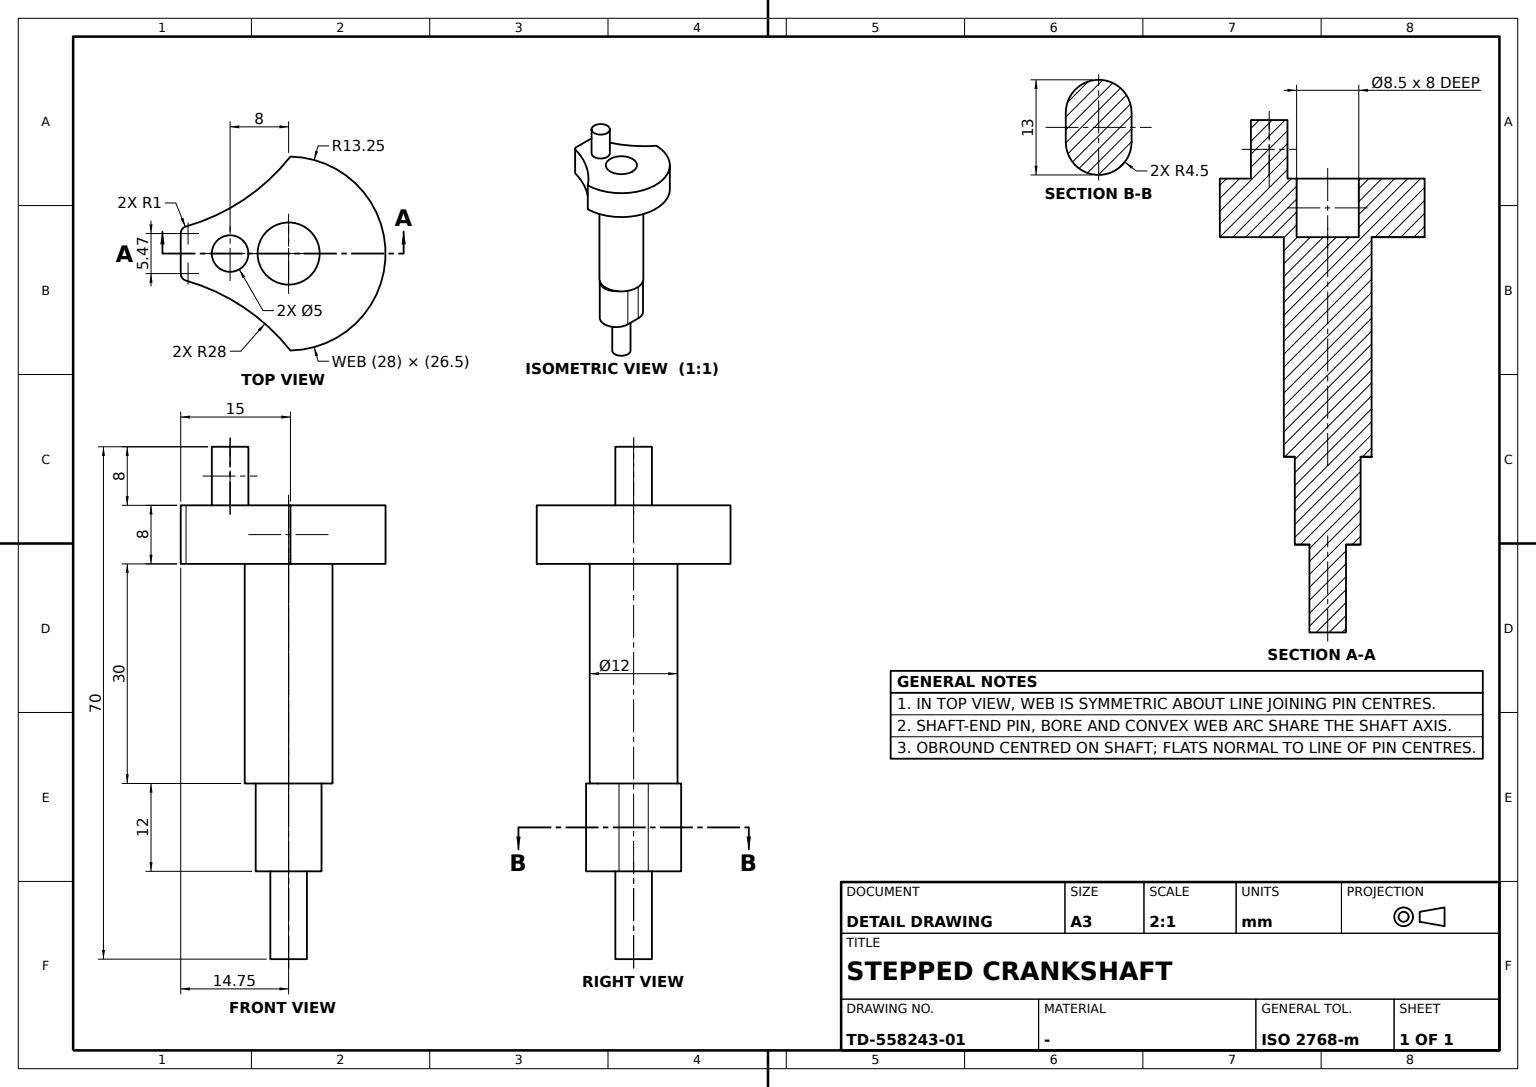
ISO-10303-21;
HEADER;
FILE_DESCRIPTION((''),'2;1');
FILE_NAME('','',(''),(''),'','','');
FILE_SCHEMA(('AUTOMOTIVE_DESIGN'));
ENDSEC;
DATA;
#1=APPLICATION_CONTEXT('');
#2=PRODUCT_CONTEXT('',#1,'mechanical');
#3=PRODUCT('','','',(#2));
#4=PRODUCT_DEFINITION_FORMATION('','',#3);
#5=PRODUCT_DEFINITION_CONTEXT('',#1,'design');
#6=PRODUCT_DEFINITION('','',#4,#5);
#7=PRODUCT_DEFINITION_SHAPE('','',#6);
#8=(LENGTH_UNIT()NAMED_UNIT(*)SI_UNIT(.MILLI.,.METRE.));
#9=(NAMED_UNIT(*)PLANE_ANGLE_UNIT()SI_UNIT($,.RADIAN.));
#10=(NAMED_UNIT(*)SI_UNIT($,.STERADIAN.)SOLID_ANGLE_UNIT());
#11=UNCERTAINTY_MEASURE_WITH_UNIT(LENGTH_MEASURE(0.005),#8,'distance_accuracy_value','');
#12=(GEOMETRIC_REPRESENTATION_CONTEXT(3)GLOBAL_UNCERTAINTY_ASSIGNED_CONTEXT((#11))GLOBAL_UNIT_ASSIGNED_CONTEXT((#8,#9,#10))REPRESENTATION_CONTEXT('',''));
#13=CARTESIAN_POINT('',(11.3410275,-4.9375,-30.));
#14=VERTEX_POINT('',#13);
#15=CARTESIAN_POINT('',(11.3410275,4.9375,-30.));
#16=VERTEX_POINT('',#15);
#17=CARTESIAN_POINT('',(14.75,0.,-30.));
#18=DIRECTION('',(0.,0.,-1.));
#19=DIRECTION('',(-1.,0.,0.));
#20=AXIS2_PLACEMENT_3D('',#17,#18,#19);
#21=CIRCLE('',#20,6.);
#22=EDGE_CURVE('',#14,#16,#21,.T.);
#23=ORIENTED_EDGE('',*,*,#22,.F.);
#24=CARTESIAN_POINT('',(18.1589725,-4.9375,-30.));
#25=VERTEX_POINT('',#24);
#26=EDGE_CURVE('',#25,#14,#21,.T.);
#27=ORIENTED_EDGE('',*,*,#26,.F.);
#28=CARTESIAN_POINT('',(18.1589725,4.9375,-30.));
#29=VERTEX_POINT('',#28);
#30=EDGE_CURVE('',#29,#25,#21,.T.);
#31=ORIENTED_EDGE('',*,*,#30,.F.);
#32=EDGE_CURVE('',#16,#29,#21,.T.);
#33=ORIENTED_EDGE('',*,*,#32,.F.);
#34=EDGE_LOOP('',(#23,#27,#31,#33));
#35=FACE_BOUND('',#34,.T.);
#36=CARTESIAN_POINT('',(20.75,0.,0.));
#37=VERTEX_POINT('',#36);
#38=CARTESIAN_POINT('',(14.75,0.,0.));
#39=DIRECTION('',(0.,0.,1.));
#40=DIRECTION('',(1.,0.,0.));
#41=AXIS2_PLACEMENT_3D('',#38,#39,#40);
#42=CIRCLE('',#41,6.);
#43=EDGE_CURVE('',#37,#37,#42,.F.);
#44=ORIENTED_EDGE('',*,*,#43,.T.);
#45=EDGE_LOOP('',(#44));
#46=FACE_BOUND('',#45,.T.);
#47=CARTESIAN_POINT('',(14.75,0.,-15.));
#48=AXIS2_PLACEMENT_3D('',#47,#18,#40);
#49=CYLINDRICAL_SURFACE('',#48,6.);
#50=ADVANCED_FACE('',(#35,#46),#49,.T.);
#51=CARTESIAN_POINT('',(19.,0.,8.));
#52=VERTEX_POINT('',#51);
#53=CARTESIAN_POINT('',(14.75,0.,8.));
#54=AXIS2_PLACEMENT_3D('',#53,#39,#40);
#55=CIRCLE('',#54,4.25);
#56=EDGE_CURVE('',#52,#52,#55,.T.);
#57=ORIENTED_EDGE('',*,*,#56,.T.);
#58=EDGE_LOOP('',(#57));
#59=FACE_BOUND('',#58,.T.);
#60=CARTESIAN_POINT('',(19.,0.,0.));
#61=VERTEX_POINT('',#60);
#62=CIRCLE('',#41,4.25);
#63=EDGE_CURVE('',#61,#61,#62,.T.);
#64=ORIENTED_EDGE('',*,*,#63,.F.);
#65=EDGE_LOOP('',(#64));
#66=FACE_BOUND('',#65,.T.);
#67=CARTESIAN_POINT('',(14.75,0.,4.));
#68=DIRECTION('',(0.,1.,0.));
#69=AXIS2_PLACEMENT_3D('',#67,#39,#68);
#70=CYLINDRICAL_SURFACE('',#69,4.25);
#71=ADVANCED_FACE('',(#59,#66),#70,.F.);
#72=CARTESIAN_POINT('',(12.25,0.,-42.));
#73=VERTEX_POINT('',#72);
#74=CARTESIAN_POINT('',(14.75,0.,-42.));
#75=AXIS2_PLACEMENT_3D('',#74,#18,#19);
#76=CIRCLE('',#75,2.5);
#77=EDGE_CURVE('',#73,#73,#76,.T.);
#78=ORIENTED_EDGE('',*,*,#77,.T.);
#79=EDGE_LOOP('',(#78));
#80=FACE_BOUND('',#79,.T.);
#81=CARTESIAN_POINT('',(12.25,0.,-54.));
#82=VERTEX_POINT('',#81);
#83=CARTESIAN_POINT('',(14.75,0.,-54.));
#84=AXIS2_PLACEMENT_3D('',#83,#18,#19);
#85=CIRCLE('',#84,2.5);
#86=EDGE_CURVE('',#82,#82,#85,.T.);
#87=ORIENTED_EDGE('',*,*,#86,.F.);
#88=EDGE_LOOP('',(#87));
#89=FACE_BOUND('',#88,.T.);
#90=CARTESIAN_POINT('',(14.75,0.,-48.));
#91=AXIS2_PLACEMENT_3D('',#90,#18,#68);
#92=CYLINDRICAL_SURFACE('',#91,2.5);
#93=ADVANCED_FACE('',(#80,#89),#92,.T.);
#94=ORIENTED_EDGE('',*,*,#63,.T.);
#95=EDGE_LOOP('',(#94));
#96=FACE_BOUND('',#95,.T.);
#97=CARTESIAN_POINT('',(0.,0.,0.));
#98=AXIS2_PLACEMENT_3D('',#97,#39,#68);
#99=PLANE('',#98);
#100=ADVANCED_FACE('',(#96),#99,.T.);
#101=CARTESIAN_POINT('',(0.7255975,3.6965592,0.));
#102=VERTEX_POINT('',#101);
#103=CARTESIAN_POINT('',(15.,13.2476413,0.));
#104=VERTEX_POINT('',#103);
#105=CARTESIAN_POINT('',(-6.9576732,30.6217769,0.));
#106=AXIS2_PLACEMENT_3D('',#105,#39,#40);
#107=CIRCLE('',#106,28.);
#108=EDGE_CURVE('',#102,#104,#107,.T.);
#109=ORIENTED_EDGE('',*,*,#108,.F.);
#110=CARTESIAN_POINT('',(0.7255975,3.6965592,8.));
#111=VERTEX_POINT('',#110);
#112=CARTESIAN_POINT('',(0.7255975,3.6965592,4.));
#113=VECTOR('',#39,1000.);
#114=LINE('',#112,#113);
#115=EDGE_CURVE('',#111,#102,#114,.F.);
#116=ORIENTED_EDGE('',*,*,#115,.F.);
#117=CARTESIAN_POINT('',(15.,13.2476413,8.));
#118=VERTEX_POINT('',#117);
#119=CARTESIAN_POINT('',(-6.9576732,30.6217769,8.));
#120=AXIS2_PLACEMENT_3D('',#119,#39,#40);
#121=CIRCLE('',#120,28.);
#122=EDGE_CURVE('',#111,#118,#121,.T.);
#123=ORIENTED_EDGE('',*,*,#122,.T.);
#124=LINE('',#103,#113);
#125=EDGE_CURVE('',#104,#118,#124,.T.);
#126=ORIENTED_EDGE('',*,*,#125,.F.);
#127=EDGE_LOOP('',(#109,#116,#123,#126));
#128=FACE_BOUND('',#127,.T.);
#129=CARTESIAN_POINT('',(-6.9576732,30.6217769,4.));
#130=AXIS2_PLACEMENT_3D('',#129,#39,#68);
#131=CYLINDRICAL_SURFACE('',#130,28.);
#132=ADVANCED_FACE('',(#128),#131,.F.);
#133=ORIENTED_EDGE('',*,*,#125,.T.);
#134=CARTESIAN_POINT('',(15.,-13.2476413,8.));
#135=VERTEX_POINT('',#134);
#136=CIRCLE('',#54,13.25);
#137=EDGE_CURVE('',#135,#118,#136,.T.);
#138=ORIENTED_EDGE('',*,*,#137,.F.);
#139=CARTESIAN_POINT('',(15.,-13.2476413,0.));
#140=VERTEX_POINT('',#139);
#141=LINE('',#139,#113);
#142=EDGE_CURVE('',#140,#135,#141,.T.);
#143=ORIENTED_EDGE('',*,*,#142,.F.);
#144=CIRCLE('',#41,13.25);
#145=EDGE_CURVE('',#140,#104,#144,.T.);
#146=ORIENTED_EDGE('',*,*,#145,.T.);
#147=EDGE_LOOP('',(#133,#138,#143,#146));
#148=FACE_BOUND('',#147,.T.);
#149=CYLINDRICAL_SURFACE('',#69,13.25);
#150=ADVANCED_FACE('',(#148),#149,.T.);
#151=ORIENTED_EDGE('',*,*,#26,.T.);
#152=CARTESIAN_POINT('',(14.75,-2.,-30.));
#153=AXIS2_PLACEMENT_3D('',#152,#18,#19);
#154=CIRCLE('',#153,4.5);
#155=EDGE_CURVE('',#25,#14,#154,.T.);
#156=ORIENTED_EDGE('',*,*,#155,.F.);
#157=EDGE_LOOP('',(#151,#156));
#158=FACE_BOUND('',#157,.T.);
#159=CARTESIAN_POINT('',(0.,0.,-30.));
#160=AXIS2_PLACEMENT_3D('',#159,#18,#40);
#161=PLANE('',#160);
#162=ADVANCED_FACE('',(#158),#161,.F.);
#163=ORIENTED_EDGE('',*,*,#43,.F.);
#164=EDGE_LOOP('',(#163));
#165=FACE_BOUND('',#164,.T.);
#166=ORIENTED_EDGE('',*,*,#108,.T.);
#167=ORIENTED_EDGE('',*,*,#145,.F.);
#168=CARTESIAN_POINT('',(0.7255975,-3.6965592,0.));
#169=VERTEX_POINT('',#168);
#170=CARTESIAN_POINT('',(-6.9576732,-30.6217769,0.));
#171=AXIS2_PLACEMENT_3D('',#170,#39,#40);
#172=CIRCLE('',#171,28.);
#173=EDGE_CURVE('',#140,#169,#172,.T.);
#174=ORIENTED_EDGE('',*,*,#173,.T.);
#175=CARTESIAN_POINT('',(0.,-2.7349442,0.));
#176=VERTEX_POINT('',#175);
#177=CARTESIAN_POINT('',(1.,-2.7349442,0.));
#178=AXIS2_PLACEMENT_3D('',#177,#39,#40);
#179=CIRCLE('',#178,1.);
#180=EDGE_CURVE('',#176,#169,#179,.T.);
#181=ORIENTED_EDGE('',*,*,#180,.F.);
#182=CARTESIAN_POINT('',(0.,2.7349442,0.));
#183=VERTEX_POINT('',#182);
#184=VECTOR('',#68,1000.);
#185=LINE('',#97,#184);
#186=EDGE_CURVE('',#176,#183,#185,.T.);
#187=ORIENTED_EDGE('',*,*,#186,.T.);
#188=CARTESIAN_POINT('',(1.,2.7349442,0.));
#189=AXIS2_PLACEMENT_3D('',#188,#39,#40);
#190=CIRCLE('',#189,1.);
#191=EDGE_CURVE('',#102,#183,#190,.T.);
#192=ORIENTED_EDGE('',*,*,#191,.F.);
#193=EDGE_LOOP('',(#166,#167,#174,#181,#187,#192));
#194=FACE_BOUND('',#193,.T.);
#195=ADVANCED_FACE('',(#165,#194),#99,.F.);
#196=CARTESIAN_POINT('',(14.75,2.,-30.));
#197=AXIS2_PLACEMENT_3D('',#196,#18,#19);
#198=CIRCLE('',#197,4.5);
#199=EDGE_CURVE('',#16,#29,#198,.T.);
#200=ORIENTED_EDGE('',*,*,#199,.F.);
#201=ORIENTED_EDGE('',*,*,#32,.T.);
#202=EDGE_LOOP('',(#200,#201));
#203=FACE_BOUND('',#202,.T.);
#204=ADVANCED_FACE('',(#203),#161,.F.);
#205=ORIENTED_EDGE('',*,*,#86,.T.);
#206=EDGE_LOOP('',(#205));
#207=FACE_BOUND('',#206,.T.);
#208=CARTESIAN_POINT('',(0.,0.,-54.));
#209=AXIS2_PLACEMENT_3D('',#208,#18,#68);
#210=PLANE('',#209);
#211=ADVANCED_FACE('',(#207),#210,.T.);
#212=CARTESIAN_POINT('',(9.25,0.,16.));
#213=VERTEX_POINT('',#212);
#214=CARTESIAN_POINT('',(6.75,0.,16.));
#215=AXIS2_PLACEMENT_3D('',#214,#39,#40);
#216=CIRCLE('',#215,2.5);
#217=EDGE_CURVE('',#213,#213,#216,.T.);
#218=ORIENTED_EDGE('',*,*,#217,.T.);
#219=EDGE_LOOP('',(#218));
#220=FACE_BOUND('',#219,.T.);
#221=CARTESIAN_POINT('',(0.,0.,16.));
#222=AXIS2_PLACEMENT_3D('',#221,#39,#40);
#223=PLANE('',#222);
#224=ADVANCED_FACE('',(#220),#223,.T.);
#225=ORIENTED_EDGE('',*,*,#56,.F.);
#226=EDGE_LOOP('',(#225));
#227=FACE_BOUND('',#226,.T.);
#228=CARTESIAN_POINT('',(0.,2.7349442,8.));
#229=VERTEX_POINT('',#228);
#230=CARTESIAN_POINT('',(1.,2.7349442,8.));
#231=AXIS2_PLACEMENT_3D('',#230,#39,#40);
#232=CIRCLE('',#231,1.);
#233=EDGE_CURVE('',#111,#229,#232,.T.);
#234=ORIENTED_EDGE('',*,*,#233,.T.);
#235=CARTESIAN_POINT('',(0.,-2.7349442,8.));
#236=VERTEX_POINT('',#235);
#237=CARTESIAN_POINT('',(0.,0.,8.));
#238=LINE('',#237,#184);
#239=EDGE_CURVE('',#236,#229,#238,.T.);
#240=ORIENTED_EDGE('',*,*,#239,.F.);
#241=CARTESIAN_POINT('',(0.7255975,-3.6965592,8.));
#242=VERTEX_POINT('',#241);
#243=CARTESIAN_POINT('',(1.,-2.7349442,8.));
#244=AXIS2_PLACEMENT_3D('',#243,#39,#40);
#245=CIRCLE('',#244,1.);
#246=EDGE_CURVE('',#236,#242,#245,.T.);
#247=ORIENTED_EDGE('',*,*,#246,.T.);
#248=CARTESIAN_POINT('',(-6.9576732,-30.6217769,8.));
#249=AXIS2_PLACEMENT_3D('',#248,#39,#40);
#250=CIRCLE('',#249,28.);
#251=EDGE_CURVE('',#135,#242,#250,.T.);
#252=ORIENTED_EDGE('',*,*,#251,.F.);
#253=ORIENTED_EDGE('',*,*,#137,.T.);
#254=ORIENTED_EDGE('',*,*,#122,.F.);
#255=EDGE_LOOP('',(#234,#240,#247,#252,#253,#254));
#256=FACE_BOUND('',#255,.T.);
#257=CARTESIAN_POINT('',(9.25,0.,8.));
#258=VERTEX_POINT('',#257);
#259=CARTESIAN_POINT('',(6.75,0.,8.));
#260=AXIS2_PLACEMENT_3D('',#259,#39,#40);
#261=CIRCLE('',#260,2.5);
#262=EDGE_CURVE('',#258,#258,#261,.T.);
#263=ORIENTED_EDGE('',*,*,#262,.F.);
#264=EDGE_LOOP('',(#263));
#265=FACE_BOUND('',#264,.T.);
#266=AXIS2_PLACEMENT_3D('',#237,#39,#68);
#267=PLANE('',#266);
#268=ADVANCED_FACE('',(#227,#256,#265),#267,.T.);
#269=ORIENTED_EDGE('',*,*,#251,.T.);
#270=CARTESIAN_POINT('',(0.7255975,-3.6965592,4.));
#271=VECTOR('',#18,1000.);
#272=LINE('',#270,#271);
#273=EDGE_CURVE('',#242,#169,#272,.T.);
#274=ORIENTED_EDGE('',*,*,#273,.T.);
#275=ORIENTED_EDGE('',*,*,#173,.F.);
#276=ORIENTED_EDGE('',*,*,#142,.T.);
#277=EDGE_LOOP('',(#269,#274,#275,#276));
#278=FACE_BOUND('',#277,.T.);
#279=CARTESIAN_POINT('',(-6.9576732,-30.6217769,4.));
#280=AXIS2_PLACEMENT_3D('',#279,#39,#68);
#281=CYLINDRICAL_SURFACE('',#280,28.);
#282=ADVANCED_FACE('',(#278),#281,.F.);
#283=CARTESIAN_POINT('',(0.,2.7349442,4.));
#284=LINE('',#283,#271);
#285=EDGE_CURVE('',#229,#183,#284,.T.);
#286=ORIENTED_EDGE('',*,*,#285,.F.);
#287=ORIENTED_EDGE('',*,*,#233,.F.);
#288=ORIENTED_EDGE('',*,*,#115,.T.);
#289=ORIENTED_EDGE('',*,*,#191,.T.);
#290=EDGE_LOOP('',(#286,#287,#288,#289));
#291=FACE_BOUND('',#290,.T.);
#292=CARTESIAN_POINT('',(1.,2.7349442,4.));
#293=AXIS2_PLACEMENT_3D('',#292,#18,#19);
#294=CYLINDRICAL_SURFACE('',#293,1.);
#295=ADVANCED_FACE('',(#291),#294,.T.);
#296=CARTESIAN_POINT('',(19.25,2.,-30.));
#297=VERTEX_POINT('',#296);
#298=CARTESIAN_POINT('',(19.25,2.,-42.));
#299=VERTEX_POINT('',#298);
#300=CARTESIAN_POINT('',(19.25,2.,-36.));
#301=LINE('',#300,#271);
#302=EDGE_CURVE('',#297,#299,#301,.T.);
#303=ORIENTED_EDGE('',*,*,#302,.F.);
#304=CARTESIAN_POINT('',(19.25,-2.,-30.));
#305=VERTEX_POINT('',#304);
#306=CARTESIAN_POINT('',(19.25,0.,-30.));
#307=LINE('',#306,#184);
#308=EDGE_CURVE('',#305,#297,#307,.T.);
#309=ORIENTED_EDGE('',*,*,#308,.F.);
#310=CARTESIAN_POINT('',(19.25,-2.,-42.));
#311=VERTEX_POINT('',#310);
#312=CARTESIAN_POINT('',(19.25,-2.,-36.));
#313=LINE('',#312,#271);
#314=EDGE_CURVE('',#305,#311,#313,.T.);
#315=ORIENTED_EDGE('',*,*,#314,.T.);
#316=CARTESIAN_POINT('',(19.25,0.,-42.));
#317=LINE('',#316,#184);
#318=EDGE_CURVE('',#311,#299,#317,.T.);
#319=ORIENTED_EDGE('',*,*,#318,.T.);
#320=EDGE_LOOP('',(#303,#309,#315,#319));
#321=FACE_BOUND('',#320,.T.);
#322=AXIS2_PLACEMENT_3D('',#304,#19,#68);
#323=PLANE('',#322);
#324=ADVANCED_FACE('',(#321),#323,.F.);
#325=ORIENTED_EDGE('',*,*,#262,.T.);
#326=EDGE_LOOP('',(#325));
#327=FACE_BOUND('',#326,.T.);
#328=ORIENTED_EDGE('',*,*,#217,.F.);
#329=EDGE_LOOP('',(#328));
#330=FACE_BOUND('',#329,.T.);
#331=CARTESIAN_POINT('',(6.75,0.,12.));
#332=AXIS2_PLACEMENT_3D('',#331,#39,#40);
#333=CYLINDRICAL_SURFACE('',#332,2.5);
#334=ADVANCED_FACE('',(#327,#330),#333,.T.);
#335=CARTESIAN_POINT('',(10.25,2.,-42.));
#336=VERTEX_POINT('',#335);
#337=CARTESIAN_POINT('',(10.25,-2.,-42.));
#338=VERTEX_POINT('',#337);
#339=CARTESIAN_POINT('',(10.25,0.,-42.));
#340=DIRECTION('',(0.,-1.,0.));
#341=VECTOR('',#340,1000.);
#342=LINE('',#339,#341);
#343=EDGE_CURVE('',#336,#338,#342,.T.);
#344=ORIENTED_EDGE('',*,*,#343,.T.);
#345=CARTESIAN_POINT('',(10.25,-2.,-30.));
#346=VERTEX_POINT('',#345);
#347=CARTESIAN_POINT('',(10.25,-2.,-36.));
#348=LINE('',#347,#271);
#349=EDGE_CURVE('',#346,#338,#348,.T.);
#350=ORIENTED_EDGE('',*,*,#349,.F.);
#351=CARTESIAN_POINT('',(10.25,2.,-30.));
#352=VERTEX_POINT('',#351);
#353=CARTESIAN_POINT('',(10.25,0.,-30.));
#354=LINE('',#353,#341);
#355=EDGE_CURVE('',#352,#346,#354,.T.);
#356=ORIENTED_EDGE('',*,*,#355,.F.);
#357=CARTESIAN_POINT('',(10.25,2.,-36.));
#358=LINE('',#357,#271);
#359=EDGE_CURVE('',#352,#336,#358,.T.);
#360=ORIENTED_EDGE('',*,*,#359,.T.);
#361=EDGE_LOOP('',(#344,#350,#356,#360));
#362=FACE_BOUND('',#361,.T.);
#363=AXIS2_PLACEMENT_3D('',#351,#40,#340);
#364=PLANE('',#363);
#365=ADVANCED_FACE('',(#362),#364,.F.);
#366=ORIENTED_EDGE('',*,*,#77,.F.);
#367=EDGE_LOOP('',(#366));
#368=FACE_BOUND('',#367,.T.);
#369=ORIENTED_EDGE('',*,*,#318,.F.);
#370=CARTESIAN_POINT('',(14.75,-2.,-42.));
#371=AXIS2_PLACEMENT_3D('',#370,#18,#19);
#372=CIRCLE('',#371,4.5);
#373=EDGE_CURVE('',#311,#338,#372,.T.);
#374=ORIENTED_EDGE('',*,*,#373,.T.);
#375=ORIENTED_EDGE('',*,*,#343,.F.);
#376=CARTESIAN_POINT('',(14.75,2.,-42.));
#377=AXIS2_PLACEMENT_3D('',#376,#18,#19);
#378=CIRCLE('',#377,4.5);
#379=EDGE_CURVE('',#336,#299,#378,.T.);
#380=ORIENTED_EDGE('',*,*,#379,.T.);
#381=EDGE_LOOP('',(#369,#374,#375,#380));
#382=FACE_BOUND('',#381,.T.);
#383=CARTESIAN_POINT('',(0.,0.,-42.));
#384=AXIS2_PLACEMENT_3D('',#383,#18,#40);
#385=PLANE('',#384);
#386=ADVANCED_FACE('',(#368,#382),#385,.T.);
#387=ORIENTED_EDGE('',*,*,#285,.T.);
#388=ORIENTED_EDGE('',*,*,#186,.F.);
#389=CARTESIAN_POINT('',(0.,-2.7349442,4.));
#390=LINE('',#389,#271);
#391=EDGE_CURVE('',#236,#176,#390,.T.);
#392=ORIENTED_EDGE('',*,*,#391,.F.);
#393=ORIENTED_EDGE('',*,*,#239,.T.);
#394=EDGE_LOOP('',(#387,#388,#392,#393));
#395=FACE_BOUND('',#394,.T.);
#396=CARTESIAN_POINT('',(0.,-3.5,0.));
#397=AXIS2_PLACEMENT_3D('',#396,#40,#68);
#398=PLANE('',#397);
#399=ADVANCED_FACE('',(#395),#398,.F.);
#400=EDGE_CURVE('',#305,#25,#154,.T.);
#401=ORIENTED_EDGE('',*,*,#400,.T.);
#402=ORIENTED_EDGE('',*,*,#155,.T.);
#403=EDGE_CURVE('',#14,#346,#154,.T.);
#404=ORIENTED_EDGE('',*,*,#403,.T.);
#405=ORIENTED_EDGE('',*,*,#349,.T.);
#406=ORIENTED_EDGE('',*,*,#373,.F.);
#407=ORIENTED_EDGE('',*,*,#314,.F.);
#408=EDGE_LOOP('',(#401,#402,#404,#405,#406,#407));
#409=FACE_BOUND('',#408,.T.);
#410=CARTESIAN_POINT('',(14.75,-2.,-36.));
#411=AXIS2_PLACEMENT_3D('',#410,#18,#40);
#412=CYLINDRICAL_SURFACE('',#411,4.5);
#413=ADVANCED_FACE('',(#409),#412,.T.);
#414=ORIENTED_EDGE('',*,*,#180,.T.);
#415=ORIENTED_EDGE('',*,*,#273,.F.);
#416=ORIENTED_EDGE('',*,*,#246,.F.);
#417=ORIENTED_EDGE('',*,*,#391,.T.);
#418=EDGE_LOOP('',(#414,#415,#416,#417));
#419=FACE_BOUND('',#418,.T.);
#420=CARTESIAN_POINT('',(1.,-2.7349442,4.));
#421=DIRECTION('',(-0.274402523,-0.961614921,0.));
#422=AXIS2_PLACEMENT_3D('',#420,#18,#421);
#423=CYLINDRICAL_SURFACE('',#422,1.);
#424=ADVANCED_FACE('',(#419),#423,.T.);
#425=EDGE_CURVE('',#352,#16,#198,.T.);
#426=ORIENTED_EDGE('',*,*,#425,.F.);
#427=ORIENTED_EDGE('',*,*,#355,.T.);
#428=ORIENTED_EDGE('',*,*,#403,.F.);
#429=ORIENTED_EDGE('',*,*,#22,.T.);
#430=EDGE_LOOP('',(#426,#427,#428,#429));
#431=FACE_BOUND('',#430,.T.);
#432=ADVANCED_FACE('',(#431),#161,.T.);
#433=ORIENTED_EDGE('',*,*,#302,.T.);
#434=ORIENTED_EDGE('',*,*,#379,.F.);
#435=ORIENTED_EDGE('',*,*,#359,.F.);
#436=ORIENTED_EDGE('',*,*,#425,.T.);
#437=ORIENTED_EDGE('',*,*,#199,.T.);
#438=EDGE_CURVE('',#29,#297,#198,.T.);
#439=ORIENTED_EDGE('',*,*,#438,.T.);
#440=EDGE_LOOP('',(#433,#434,#435,#436,#437,#439));
#441=FACE_BOUND('',#440,.T.);
#442=CARTESIAN_POINT('',(14.75,2.,-36.));
#443=AXIS2_PLACEMENT_3D('',#442,#18,#40);
#444=CYLINDRICAL_SURFACE('',#443,4.5);
#445=ADVANCED_FACE('',(#441),#444,.T.);
#446=ORIENTED_EDGE('',*,*,#438,.F.);
#447=ORIENTED_EDGE('',*,*,#30,.T.);
#448=ORIENTED_EDGE('',*,*,#400,.F.);
#449=ORIENTED_EDGE('',*,*,#308,.T.);
#450=EDGE_LOOP('',(#446,#447,#448,#449));
#451=FACE_BOUND('',#450,.T.);
#452=ADVANCED_FACE('',(#451),#161,.T.);
#453=CLOSED_SHELL('',(#50,#71,#93,#100,#132,#150,#162,#195,#204,#211,#224,#268,#282,#295,#324,#334,#365,#386,#399,#413,#424,#432,#445,#452));
#454=MANIFOLD_SOLID_BREP('',#453);
#455=ADVANCED_BREP_SHAPE_REPRESENTATION('',(#454),#12);
#456=SHAPE_DEFINITION_REPRESENTATION(#7,#455);
ENDSEC;
END-ISO-10303-21;
